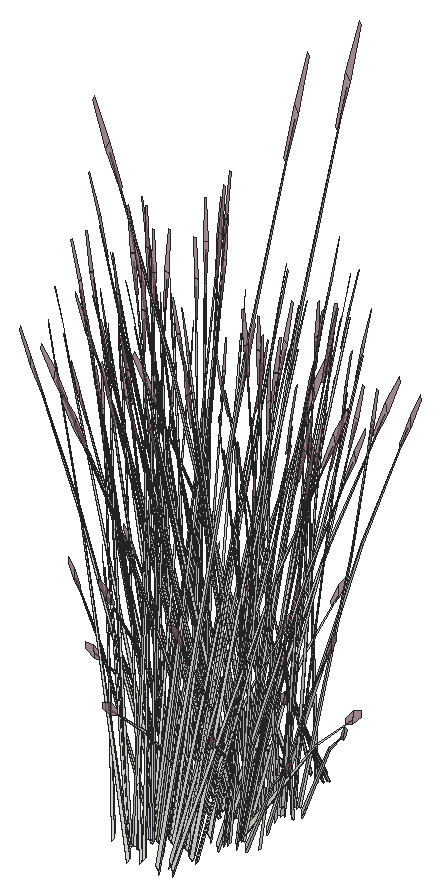
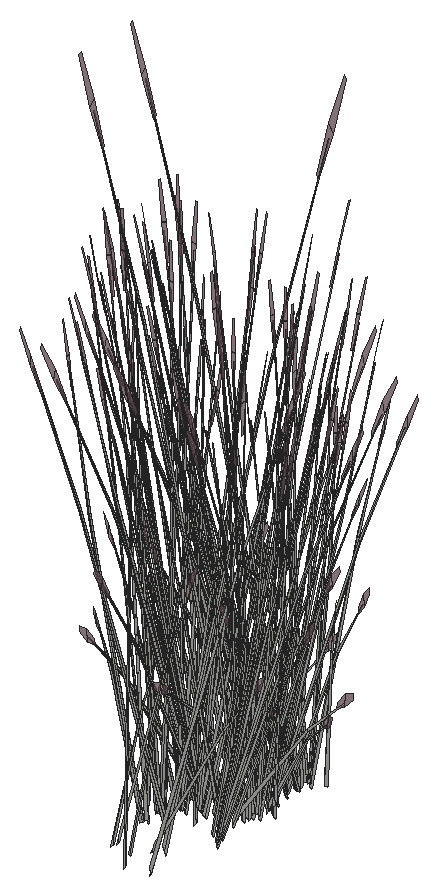
# SketchUp Ruby script. Lengths in inches.
U = 1.inch
M = Sketchup.active_model
def pt(a) = Geom::Point3d.new(a.map { |v| v * U })
def face(e, loops, mat)
  f = e.add_face(loops[0].map { |a| pt(a) })
  loops[1..].each { |l| e.add_face(l.map { |a| pt(a) }).erase! }
  f.material = f.back_material = mat if mat
  f
end
# faces: each face lists its corners as indices into pts; further lists are holes
def faces(e, pts, list, mat = nil) = list.each { |f| face(e, (f[0].is_a?(Array) ? f : [f]).map { |l| l.map { |i| pts[i] } }, mat) }
# xy, xz, yz: faces in a plane at the given z, y or x. An outline is a flat list of corners, or four numbers for a rectangle; further outlines are holes
def ring(l) = l.size == 4 ? [[l[0], l[1]], [l[2], l[1]], [l[2], l[3]], [l[0], l[3]]] : l.each_slice(2).to_a
def flat(e, list, mat, &to3) = list.each { |f| face(e, (f[0].is_a?(Array) ? f : [f]).map { |l| ring(l).map { |u, v| to3.(u, v) } }, mat) }
def xy(e, z, list, mat = nil) = flat(e, list, mat) { |x, y| [x, y, z] }
def xz(e, y, list, mat = nil) = flat(e, list, mat) { |x, z| [x, y, z] }
def yz(e, x, list, mat = nil) = flat(e, list, mat) { |y, z| [x, y, z] }
def lines(e, pts, list) = list.each { |a, b| e.add_line(pt(pts[a]), pt(pts[b])) }
# prism: a flat outline (further loops are holes) pulled along v
def prism(e, loops, v, mat = nil)
  f = face(e, loops, mat); d = Geom::Vector3d.new(v.map { |x| x * U })
  f.pushpull(f.normal.samedirection?(d) ? d.length : -d.length)
end
def box(e, o, s, mat = nil) = prism(e, [[o, [o[0] + s[0], o[1], o[2]], [o[0] + s[0], o[1] + s[1], o[2]], [o[0], o[1] + s[1], o[2]]]], [0, 0, s[2]], mat)
def at(x, y, z, deg = 0) = Geom::Transformation.translation(pt([x, y, z])) * Geom::Transformation.rotation(ORIGIN, Z_AXIS, deg.degrees)
def axes(o, x, y, z) = Geom::Transformation.new([*x, 0, *y, 0, *z, 0, *pt(o).to_a, 1])
def part(name) = M.definitions.add(name)
# library, detail: a bought-in or finely detailed component or shape, given as its bounding box
def library(name, o, s) = part(name).tap { |d| box(d.entities, o, s) }
def detail(e, o, s) = box(e.add_group.entities, o, s)
def put(e, d, t, mat = nil) = e.add_instance(d, t).tap { |i| i.material = mat if mat }
def group(e, t, mat = nil) = e.add_group.tap { |g| g.transformation = t; g.material = mat if mat }.entities
root = M.entities
M.materials.add("LightPink_Translucent").color = [144, 107, 117]
M.materials["LightPink_Translucent"].alpha = 0.75
c1 = part("blade")
p = [[2.15,0.21,22],[0,0.17,0],[0.09,0.45,0],[2.18,0.31,22],[2.29,0.31,22],[0.38,0.45,0],
  [2.48,0.24,33],[2.49,0.24,33],[2.48,0.22,33]]
faces(c1.entities,p,[[0,1,2,3],[4,5,2,3],[6,3,4,7],[8,0,3,6]])
c2 = part("seeds")
p = [[0.3,-0.1,1.38],[-0.01,-0.03,1.59],[-0.01,-0.03,0.03],[0.14,-0.07,-0.07],[0.29,-0.03,3],[0.15,0.01,3.11]]
faces(c2.entities,p,[[0,1,2,3],[1,0,4,5]],"LightPink_Translucent")
c3 = part("blade with seeds")
put(c3.entities,c1,at(0,0,0))
put(c3.entities,c2,axes([2.4,0.25,30.99],[1.5799,-0.05474,1.17369],[-0.12525,1.92788,0.29478],[-0.07173,-0.02425,1.56792]))
put(root,c3,axes([427.19,466.05,154],[-0.28133,-0.19836,0.05432],[0.16379,-0.28248,0.42765],[-0.0902,0.09132,0.65209]))
put(root,c3,axes([427.32,465.53,153.27],[0.14219,-0.09977,1.44779],[0.11971,0.461,0.11706],[-0.22323,0.10419,0.61892]))
put(root,c3,axes([431.01,468.83,154],[0.28133,0.19836,0.05432],[-0.16379,0.28248,0.42765],[0.0902,-0.09132,0.65209]))
put(root,c3,axes([430.93,468.75,154],[0.10163,0.43409,0.40553],[-0.39868,0.07534,0.33437],[0.1175,-0.10209,0.83914]))
put(root,c3,axes([432.01,469.28,153.98],[0.05687,-0.07184,1.47793],[-0.07279,-0.44069,-0.23373],[0.14268,-0.08356,0.11853]))
put(root,c3,axes([427.2,467.56,153.98],[0.03038,0.04707,1.49853],[-0.14646,0.42312,-0.1416],[-0.14833,0.00306,0.26519]))
put(root,c3,axes([428.2,471.875,153.27],[0.09368,0.15143,1.44779],[-0.43286,0.12749,0.11706],[-0.09783,-0.23774,0.61892]))
put(root,c3,axes([426.14,465.82,153.98],[0.0523,0.01265,1.49853],[0.16179,0.41674,-0.1416],[-0.10706,0.10938,0.26519]))
put(root,c3,axes([428.91,470.87,153.98],[-0.06268,-0.06613,1.47793],[-0.4183,0.04193,-0.23373],[-0.06676,-0.15817,0.11853]))
put(root,c3,axes([427.625,468.43,153.95],[-0.29757,0.31243,-0.43168],[-0.2606,-0.33005,-0.33437],[-0.15119,-0.04754,0.82598]))
put(root,c3,axes([430.69,466.75,153.82],[0.23317,0.29531,-0.29918],[-0.26625,0.27955,0.38624],[0.13527,0.04253,0.73904]))
put(root,c3,axes([430.57,466.86,154],[-0.02064,0.35866,0.05432],[-0.3116,-0.00983,0.42765],[0.11936,0.03753,0.65209]))
put(root,c3,axes([427.23,466.22,153.82],[-0.35672,0.06741,-0.29918],[-0.09419,-0.38534,0.38624],[-0.10222,0.1035,0.73904]))
put(root,c3,axes([430.6,466.75,154],[-0.30217,0.31079,0.40553],[-0.2606,-0.33005,0.33437],[0.14177,0.05733,0.83914]))
put(root,c3,axes([427.78,468.11,154.25],[-0.02194,0.47967,-0.10273],[-0.41546,-0.01311,-0.57019],[-0.16001,-0.03332,0.8664]))
put(root,c3,axes([430.89,469.95,154.25],[-0.20619,-0.42709,-0.10273],[0.36595,-0.20988,-0.57019],[0.15422,-0.05635,0.8664]))
put(root,c3,axes([430.87,469.58,153.95],[0.11102,-0.42903,-0.43168],[0.38064,0.14706,-0.33437],[0.15325,-0.03934,0.82598]))
put(root,c3,axes([427.25,468.77,153.27],[0.16998,-0.01068,1.44779],[-0.11276,0.46299,0.11706],[-0.24224,-0.02864,0.61892]))
put(root,c3,axes([430.79,471.68,153.98],[-0.00396,-0.09387,1.47793],[-0.33411,-0.2713,-0.23373],[0.05166,-0.16446,0.11853]))
put(root,c3,axes([429.39,471.66,153.82],[0.12355,-0.36271,-0.29918],[0.36044,0.10579,0.38624],[-0.03305,-0.14603,0.73904]))
put(root,c3,axes([429.66,472.14,153.27],[-0.0763,0.16212,1.44779],[-0.3201,-0.3355,0.11706],[0.1444,-0.2091,0.61892]))
put(root,c3,axes([430.7,471.35,153.98],[-0.04162,0.03603,1.49853],[-0.40776,-0.12155,-0.1416],[-0.01476,-0.15722,0.26519]))
put(root,c3,axes([429.86,465.99,153.27],[-0.15222,-0.08126,1.44779],[0.31502,-0.34091,0.11706],[0.19634,0.15379,0.61892]))
put(root,c3,axes([429.88,464.92,153.78],[-0.35411,-0.24507,1.16821],[0.37391,-0.38156,0.50405],[0.11425,0.22994,1.12919]))
put(root,c3,axes([429.21,471.91,153.95],[-0.40284,-0.11824,-0.43168],[0.13808,-0.40538,-0.33437],[-0.03694,-0.16321,0.82598]))
put(root,c3,axes([427.33,465.95,154.25],[0.37908,0.26007,-0.10273],[-0.21839,0.37663,-0.57019],[-0.1071,0.13092,0.8664]))
put(root,c3,axes([430.08,472.22,153.95],[-0.29336,-0.31691,-0.43168],[0.3099,-0.27755,-0.33437],[0.04464,-0.16102,0.82598]))
put(root,c3,axes([429.61,467.3,154.25],[0.2442,-0.40372,-0.10273],[0.35364,0.23259,-0.57019],[0.12293,0.11406,0.8664]))
put(root,c3,axes([428.49,470.65,153.98],[-0.00765,0.05653,1.49853],[-0.37706,0.20517,-0.1416],[-0.11096,-0.10488,0.26519]))
put(root,c3,axes([427.84,465.84,153.27],[0.10236,-0.14492,1.44779],[0.25844,0.39118,0.11706],[-0.17726,0.17814,0.61892]))
put(root,c3,axes([427.18,469.12,154],[0.11578,-0.43006,0.40553],[0.38064,0.14706,0.33437],[-0.14969,0.02584,0.83914]))
put(root,c3,axes([427.52,466.26,153.95],[0.10528,0.43067,-0.43168],[-0.39868,0.07534,-0.33437],[-0.11425,0.11568,0.82598]))
put(root,c3,axes([427.15,469,154],[-0.15051,-0.3216,0.05432],[0.27447,-0.15741,0.42765],[-0.12099,0.03106,0.65209]))
put(root,c3,axes([429.43,471.75,154],[0.4038,0.12331,0.40553],[-0.13808,0.40538,0.33437],[-0.02427,-0.15942,0.83914]))
put(root,c3,axes([429.29,467.64,153.98],[0.00121,-0.0571,1.49853],[0.35119,-0.25193,-0.1416],[0.12199,0.08992,0.26519]))
put(root,c3,axes([429.55,471.89,154.25],[-0.40102,0.2196,-0.10273],[-0.19707,-0.38974,-0.57019],[-0.05291,-0.16424,0.8664]))
put(root,c3,axes([430.38,472.39,154.25],[-0.45039,-0.02337,-0.10273],[0.01231,-0.44247,-0.57019],[0.03129,-0.17041,0.8664]))
put(root,c3,axes([427.75,466.98,154],[-0.33677,-0.02198,0.05432],[0.00923,-0.33185,0.42765],[-0.03524,0.12712,0.65209]))
put(root,c3,axes([430.35,472.1,153.82],[0.27728,-0.24833,-0.29918],[0.26248,0.28355,0.38624],[0.03994,-0.14407,0.73904]))
put(root,c3,axes([429.54,471.72,154],[0.30197,-0.1603,0.05432],[0.1478,0.29231,0.42765],[-0.02916,-0.12885,0.65209]))
put(root,c3,axes([427.85,467.01,154],[-0.29182,-0.32181,0.40553],[0.3099,-0.27755,0.33437],[-0.05383,0.15098,0.83914]))
put(root,c3,axes([429.9,467.1,153.95],[0.40438,-0.11212,-0.43168],[0.07074,0.4246,-0.33437],[0.10862,0.12168,0.82598]))
put(root,c3,axes([428.35,471.8,153.82],[-0.06329,-0.37991,-0.29918],[0.36182,-0.10032,0.38624],[-0.09718,-0.10887,0.73904]))
put(root,c3,axes([431.1,469.78,153.82],[0.34057,0.13158,-0.29918],[-0.09933,0.38387,0.38624],[0.13712,-0.0352,0.73904]))
put(root,c3,axes([427.1,469.16,153.82],[-0.34057,-0.13158,-0.29918],[0.09933,-0.38387,0.38624],[-0.13712,0.0352,0.73904]))
put(root,c3,axes([429.7,467.45,154],[-0.18625,0.29962,0.05432],[-0.26523,-0.17444,0.42765],[0.08575,0.09606,0.65209]))
put(root,c3,axes([428.51,471.76,154],[0.18625,-0.29962,0.05432],[0.26523,0.17444,0.42765],[-0.08575,-0.09606,0.65209]))
put(root,c3,axes([429.78,467.37,154],[-0.4076,0.10824,0.40553],[-0.07074,-0.4246,0.33437],[0.09586,0.12514,0.83914]))
put(root,c3,axes([430.18,469.3,153.27],[-0.16998,0.01068,1.44779],[0.11276,-0.46299,0.11706],[0.24224,0.02864,0.61892]))
put(root,c3,axes([427.57,472.35,153.27],[0.15222,0.08126,1.44779],[-0.31502,0.34091,0.11706],[-0.19634,-0.15379,0.61892]))
put(root,c3,axes([427.77,466.2,153.27],[0.0763,-0.16212,1.44779],[0.3201,0.3355,0.11706],[-0.1444,0.2091,0.61892]))
put(root,c3,axes([431.05,469.9375,154],[0.15051,0.3216,0.05432],[-0.27447,0.15741,0.42765],[0.12099,-0.03106,0.65209]))
put(root,c3,axes([431.03,469.82,154],[-0.11578,0.43006,0.40553],[-0.38064,-0.14706,0.33437],[0.14969,-0.02584,0.83914]))
put(root,c3,axes([428.31,472.11,153.95],[-0.40438,0.11212,-0.43168],[-0.07074,-0.4246,-0.33437],[-0.10862,-0.12168,0.82598]))
put(root,c3,axes([430.35,472.2,154],[0.29182,0.32181,0.40553],[-0.3099,0.27755,0.33437],[0.05383,-0.15098,0.83914]))
put(root,c3,axes([428.66,467.49,154],[-0.30197,0.1603,0.05432],[-0.1478,-0.29231,0.42765],[0.02916,0.12885,0.65209]))
put(root,c3,axes([428.59,471.73,154.59],[-0.2735,0.45217,-0.11506],[-0.39608,-0.2605,-0.63862],[-0.13768,-0.12775,0.97037]))
put(root,c3,axes([427.85,467.11,153.82],[-0.27728,0.24833,-0.29918],[-0.26248,-0.28355,0.38624],[-0.03994,0.14407,0.73904]))
put(root,c3,axes([426.9,467.04,153.98],[-0.01019,0.09334,1.47793],[0.28908,0.3247,-0.23373],[-0.07568,0.15355,0.11853]))
put(root,c3,axes([430.46,472.23,154],[0.33677,0.02198,0.05432],[-0.00923,0.33185,0.42765],[0.03524,-0.12712,0.65209]))
put(root,c3,axes([427.82,466.83,154.56],[0.45039,0.02337,-0.11403],[-0.01231,0.44247,-0.63292],[-0.03129,0.17041,0.9617]))
put(root,c3,axes([428.66,467.32,154.25],[0.40102,-0.2196,-0.10273],[0.19707,0.38974,-0.57019],[0.05291,0.16424,0.8664]))
put(root,c3,axes([430.6875,472.95,153.95],[-0.10528,-0.43067,-0.43168],[0.39868,-0.07534,-0.33437],[0.11425,-0.11568,0.82598]))
put(root,c3,axes([428.14,469.1,152.82],[0.11649,-0.06823,1.49584],[0.04017,0.47639,0.11706],[-0.25231,0.06321,0.53462]))
put(root,c3,axes([428.13,466.99,154.23],[0.29336,0.31691,-0.47917],[-0.3099,0.27755,-0.37115],[-0.04464,0.16102,0.91684]))
put(root,c3,axes([427.54,471.6,153.98],[-0.08817,-0.00333,1.47793],[-0.28072,0.33293,-0.23373],[-0.14978,-0.06803,0.11853]))
put(root,c3,axes([430.875,473.26,154.25],[-0.37908,-0.26007,-0.10273],[0.21839,-0.37663,-0.57019],[0.1071,-0.13092,0.8664]))
put(root,c3,axes([429,467.3,153.95],[0.40284,0.11824,-0.43168],[-0.13808,0.40538,-0.33437],[0.03694,0.16321,0.82598]))
put(root,c3,axes([429.23,466.46,153.27],[-0.09368,-0.15143,1.44779],[0.43286,-0.12749,0.11706],[0.09783,0.23774,0.61892]))
put(root,c3,axes([431.71,471.21,153.98],[-0.03706,-0.04129,1.49853],[0.08106,-0.44261,-0.1416],[0.14596,-0.02828,0.26519]))
put(root,c3,axes([429.31,474.68,152.81],[0.35414,0.19019,1.27785],[-0.34693,0.40974,0.50532],[-0.1554,-0.24285,1.07126]))
put(root,c3,axes([426.89,469.42,153.98],[-0.06692,0.06124,1.47793],[0.00569,0.44742,-0.23373],[-0.15339,0.05818,0.11853]))
put(root,c3,axes([427.34,469.36,153.95],[-0.11102,0.42903,-0.43168],[-0.38064,-0.14706,-0.33437],[-0.15325,0.03934,0.82598]))
put(root,c3,axes([427.32,468.99,154.25],[0.20619,0.42709,-0.10273],[-0.36595,0.20988,-0.57019],[-0.15422,0.05635,0.8664]))
put(root,c3,axes([428.82,467.55,153.82],[-0.12355,0.36271,-0.29918],[-0.36044,-0.10579,0.38624],[0.03305,0.14603,0.73904]))
put(root,c3,axes([431.39,470.85,153.32],[-0.07843,-0.39649,-0.0295],[0.37072,-0.09115,-0.13375],[0.07742,0.02514,0.44114]))
put(root,c3,axes([430.43,470.83,154.25],[0.02194,-0.47967,-0.10273],[0.41546,0.01311,-0.57019],[0.16001,0.03332,0.8664]))
put(root,c3,axes([431.81,473.14,153.98],[-0.05353,-0.00358,1.49853],[-0.22227,-0.38383,-0.1416],[0.08926,-0.1262,0.26519]))
put(root,c3,axes([428.04,466.85,154.51],[-0.01066,0.43628,-0.66621],[-0.44902,-0.0293,0.0804],[-0.04739,0.18483,0.94242]))
put(root,c3,axes([426.87,467.99,153.98],[0.04649,-0.02848,1.49853],[0.38427,0.18941,-0.1416],[-0.00903,0.15771,0.26519]))
put(root,c3,axes([428.46,466.54,153.27],[-0.01003,-0.18103,1.44779],[0.43473,0.12009,0.11706],[-0.02689,0.25798,0.61892]))
put(root,c3,axes([430.98,472.99,153.82],[0.35672,-0.06741,-0.29918],[0.09419,0.38534,0.38624],[0.10222,-0.1035,0.73904]))
put(root,c3,axes([427.63,472.35,154],[0.02064,-0.35866,0.05432],[0.3116,0.00983,0.42765],[-0.11936,-0.03753,0.65209]))
put(root,c3,axes([427.51,472.46,153.82],[-0.23317,-0.29531,-0.29918],[0.26625,-0.27955,0.38624],[-0.13527,-0.04253,0.73904]))
put(root,c3,axes([430.79,470.55,153.98],[0.08791,-0.00798,1.47793],[0.24113,-0.36643,-0.23373],[0.15637,0.04837,0.11853]))
put(root,c3,axes([428.5625,468.19,153.98],[0.05195,0.07595,1.47793],[0.41921,0.02984,-0.23373],[0.04216,0.1675,0.11853]))
put(root,c3,axes([427.27,470.1875,154],[-0.10163,-0.43409,0.40553],[0.39868,-0.07534,0.33437],[-0.1175,0.10209,0.83914]))
put(root,c3,axes([427.19,470.1,154],[-0.28133,-0.19836,0.05432],[0.16379,-0.28248,0.42765],[-0.0902,0.09132,0.65209]))
put(root,c3,axes([427.32,469.58,153.27],[0.14219,-0.09977,1.44779],[0.11971,0.461,0.11706],[-0.22323,0.10419,0.61892]))
put(root,c3,axes([427.89,467.46,152.84],[0.009,-0.24349,1.30391],[0.40497,0.12861,0.18019],[-0.03509,0.2595,0.61571]))
put(root,c3,axes([431.01,473.16,154],[0.28133,0.19836,0.05432],[-0.16379,0.28248,0.42765],[0.0902,-0.09132,0.65209]))
put(root,c3,axes([430.93,473.08,154],[0.10163,0.43409,0.40553],[-0.39868,0.07534,0.33437],[0.1175,-0.10209,0.83914]))
put(root,c3,axes([432.01,473.6,153.98],[0.05687,-0.07184,1.47793],[-0.07279,-0.44069,-0.23373],[0.14268,-0.08356,0.11853]))
put(root,c3,axes([426.14,469.87,153.98],[0.0523,0.01265,1.49853],[0.16179,0.41674,-0.1416],[-0.10706,0.10938,0.26519]))
put(root,c3,axes([430.69,470.8,153.82],[0.23317,0.29531,-0.29918],[-0.26625,0.27955,0.38624],[0.13527,0.04253,0.73904]))
put(root,c3,axes([427.2,471.88,153.98],[0.03038,0.04707,1.49853],[-0.14646,0.42312,-0.1416],[-0.14833,0.00306,0.26519]))
put(root,c3,axes([430.57,470.91,154],[-0.02064,0.35866,0.05432],[-0.3116,-0.00983,0.42765],[0.11936,0.03753,0.65209]))
put(root,c3,axes([427.23,470.27,153.82],[-0.35672,0.06741,-0.29918],[-0.09419,-0.38534,0.38624],[-0.10222,0.1035,0.73904]))
put(root,c3,axes([430.6,470.8,154],[-0.30217,0.31079,0.40553],[-0.2606,-0.33005,0.33437],[0.14177,0.05733,0.83914]))
put(root,c3,axes([427.625,472.76,153.95],[-0.29757,0.31243,-0.43168],[-0.2606,-0.33005,-0.33437],[-0.15119,-0.04754,0.82598]))
put(root,c3,axes([427.78,472.43,154.25],[-0.02194,0.47967,-0.10273],[-0.41546,-0.01311,-0.57019],[-0.16001,-0.03332,0.8664]))
put(root,c3,axes([430.89,474.27,154.25],[-0.20619,-0.42709,-0.10273],[0.36595,-0.20988,-0.57019],[0.15422,-0.05635,0.8664]))
put(root,c3,axes([430.87,473.9,153.95],[0.11102,-0.42903,-0.43168],[0.38064,0.14706,-0.33437],[0.15325,-0.03934,0.82598]))
put(root,c3,axes([429.86,470.04,153.27],[-0.15222,-0.08126,1.44779],[0.31502,-0.34091,0.11706],[0.19634,0.15379,0.61892]))
put(root,c3,axes([427.25,473.09,153.27],[0.16998,-0.01068,1.44779],[-0.11276,0.46299,0.11706],[-0.24224,-0.02864,0.61892]))
put(root,c3,axes([429.88,468.97,153.78],[-0.35411,-0.24507,1.16821],[0.37391,-0.38156,0.50405],[0.11425,0.22994,1.12919]))
put(root,c3,axes([427.33,470.01,154.25],[0.37908,0.26007,-0.10273],[-0.21839,0.37663,-0.57019],[-0.1071,0.13092,0.8664]))
put(root,c3,axes([429.61,471.36,154.25],[0.2442,-0.40372,-0.10273],[0.35364,0.23259,-0.57019],[0.12293,0.11406,0.8664]))
put(root,c3,axes([427.84,469.89,153.27],[0.10236,-0.14492,1.44779],[0.25844,0.39118,0.11706],[-0.17726,0.17814,0.61892]))
put(root,c3,axes([427.52,470.32,153.95],[0.10528,0.43067,-0.43168],[-0.39868,0.07534,-0.33437],[-0.11425,0.11568,0.82598]))
put(root,c3,axes([429.29,471.69,153.98],[0.00121,-0.0571,1.49853],[0.35119,-0.25193,-0.1416],[0.12199,0.08992,0.26519]))
put(root,c3,axes([427.75,471.04,154],[-0.33677,-0.02198,0.05432],[0.00923,-0.33185,0.42765],[-0.03524,0.12712,0.65209]))
put(root,c3,axes([427.85,471.07,154],[-0.29182,-0.32181,0.40553],[0.3099,-0.27755,0.33437],[-0.05383,0.15098,0.83914]))
put(root,c3,axes([429.9,471.16,153.95],[0.40438,-0.11212,-0.43168],[0.07074,0.4246,-0.33437],[0.10862,0.12168,0.82598]))
put(root,c3,axes([427.18,473.44,154],[0.11578,-0.43006,0.40553],[0.38064,0.14706,0.33437],[-0.14969,0.02584,0.83914]))
put(root,c3,axes([428.2,477.41,153.27],[0.09368,0.15143,1.44779],[-0.43286,0.12749,0.11706],[-0.09783,-0.23774,0.61892]))
put(root,c3,axes([427.15,473.33,154],[-0.15051,-0.3216,0.05432],[0.27447,-0.15741,0.42765],[-0.12099,0.03106,0.65209]))
put(root,c3,axes([428.91,476.41,153.98],[-0.06268,-0.06613,1.47793],[-0.4183,0.04193,-0.23373],[-0.06676,-0.15817,0.11853]))
put(root,c3,axes([429.7,471.5,154],[-0.18625,0.29962,0.05432],[-0.26523,-0.17444,0.42765],[0.08575,0.09606,0.65209]))
put(root,c3,axes([431.1,474.1,153.82],[0.34057,0.13158,-0.29918],[-0.09933,0.38387,0.38624],[0.13712,-0.0352,0.73904]))
put(root,c3,axes([429.78,471.42,154],[-0.4076,0.10824,0.40553],[-0.07074,-0.4246,0.33437],[0.09586,0.12514,0.83914]))
put(root,c3,axes([427.1,473.49,153.82],[-0.34057,-0.13158,-0.29918],[0.09933,-0.38387,0.38624],[-0.13712,0.0352,0.73904]))
put(root,c3,axes([427.77,470.25,153.27],[0.0763,-0.16212,1.44779],[0.3201,0.3355,0.11706],[-0.1444,0.2091,0.61892]))
put(root,c3,axes([430.79,477.22,153.98],[-0.00396,-0.09387,1.47793],[-0.33411,-0.2713,-0.23373],[0.05166,-0.16446,0.11853]))
put(root,c3,axes([428.66,471.55,154],[-0.30197,0.1603,0.05432],[-0.1478,-0.29231,0.42765],[0.02916,0.12885,0.65209]))
put(root,c3,axes([429.39,477.2,153.82],[0.12355,-0.36271,-0.29918],[0.36044,0.10579,0.38624],[-0.03305,-0.14603,0.73904]))
put(root,c3,axes([429.66,477.68,153.27],[-0.0763,0.16212,1.44779],[-0.3201,-0.3355,0.11706],[0.1444,-0.2091,0.61892]))
put(root,c3,axes([430.7,476.88,153.98],[-0.04162,0.03603,1.49853],[-0.40776,-0.12155,-0.1416],[-0.01476,-0.15722,0.26519]))
put(root,c3,axes([430.18,473.625,153.27],[-0.16998,0.01068,1.44779],[0.11276,-0.46299,0.11706],[0.24224,0.02864,0.61892]))
put(root,c3,axes([427.85,471.16,153.82],[-0.27728,0.24833,-0.29918],[-0.26248,-0.28355,0.38624],[-0.03994,0.14407,0.73904]))
